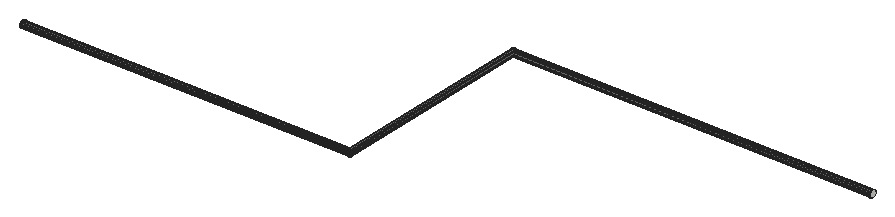
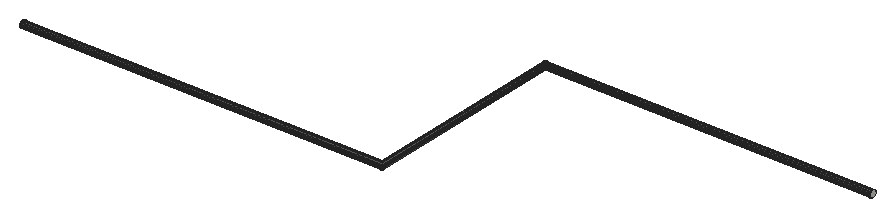
# SketchUp Ruby script. Lengths in inches.
U = 1.inch
M = Sketchup.active_model
def pt(a) = Geom::Point3d.new(a.map { |v| v * U })
def face(e, loops, mat)
  f = e.add_face(loops[0].map { |a| pt(a) })
  loops[1..].each { |l| e.add_face(l.map { |a| pt(a) }).erase! }
  f.material = f.back_material = mat if mat
  f
end
# faces: each face lists its corners as indices into pts; further lists are holes
def faces(e, pts, list, mat = nil) = list.each { |f| face(e, (f[0].is_a?(Array) ? f : [f]).map { |l| l.map { |i| pts[i] } }, mat) }
# xy, xz, yz: faces in a plane at the given z, y or x. An outline is a flat list of corners, or four numbers for a rectangle; further outlines are holes
def ring(l) = l.size == 4 ? [[l[0], l[1]], [l[2], l[1]], [l[2], l[3]], [l[0], l[3]]] : l.each_slice(2).to_a
def flat(e, list, mat, &to3) = list.each { |f| face(e, (f[0].is_a?(Array) ? f : [f]).map { |l| ring(l).map { |u, v| to3.(u, v) } }, mat) }
def xy(e, z, list, mat = nil) = flat(e, list, mat) { |x, y| [x, y, z] }
def xz(e, y, list, mat = nil) = flat(e, list, mat) { |x, z| [x, y, z] }
def yz(e, x, list, mat = nil) = flat(e, list, mat) { |y, z| [x, y, z] }
def lines(e, pts, list) = list.each { |a, b| e.add_line(pt(pts[a]), pt(pts[b])) }
# prism: a flat outline (further loops are holes) pulled along v
def prism(e, loops, v, mat = nil)
  f = face(e, loops, mat); d = Geom::Vector3d.new(v.map { |x| x * U })
  f.pushpull(f.normal.samedirection?(d) ? d.length : -d.length)
end
def box(e, o, s, mat = nil) = prism(e, [[o, [o[0] + s[0], o[1], o[2]], [o[0] + s[0], o[1] + s[1], o[2]], [o[0], o[1] + s[1], o[2]]]], [0, 0, s[2]], mat)
def at(x, y, z, deg = 0) = Geom::Transformation.translation(pt([x, y, z])) * Geom::Transformation.rotation(ORIGIN, Z_AXIS, deg.degrees)
def axes(o, x, y, z) = Geom::Transformation.new([*x, 0, *y, 0, *z, 0, *pt(o).to_a, 1])
def part(name) = M.definitions.add(name)
# library, detail: a bought-in or finely detailed component or shape, given as its bounding box
def library(name, o, s) = part(name).tap { |d| box(d.entities, o, s) }
def detail(e, o, s) = box(e.add_group.entities, o, s)
def put(e, d, t, mat = nil) = e.add_instance(d, t).tap { |i| i.material = mat if mat }
def group(e, t, mat = nil) = e.add_group.tap { |g| g.transformation = t; g.material = mat if mat }.entities
root = M.entities
M.materials.add("[Color M05]").color = [114, 114, 114]
yz(root,18,[[228,288.3125,227.74,288.34,227.5,288.44,227.29,288.6,227.13,288.8125,227.03,289.05,227,289.3125,227.03,289.57,227.13,289.8125,227.29,290.02,227.5,290.18,227.74,290.28,228,290.3125,228.26,290.28,228.5,290.18,228.71,290.02,228.87,289.8125,228.97,289.57,229,289.3125,228.97,289.05,228.87,288.8125,228.71,288.6,228.5,288.44,228.26,288.34]])
yz(root,231,[[291,288.3125,291.26,288.34,291.5,288.44,291.71,288.6,291.87,288.8125,291.97,289.05,292,289.3125,291.97,289.57,291.87,289.8125,291.71,290.02,291.5,290.18,291.26,290.28,291,290.3125,290.74,290.28,290.5,290.18,290.29,290.02,290.13,289.8125,290.03,289.57,290,289.3125,290.03,289.05,290.13,288.8125,290.29,288.6,290.5,288.44,290.74,288.34]])
p = [[119.76,227.74,288.34],[120,227.5,288.44],[18,227.5,288.44],[18,227.74,288.34],[119.76,290.74,288.34],[120,290.5,288.44],
  [119.5,228,288.3125],[18,228,288.3125],[119.5,291,288.3125],[119.24,228.26,288.34],[18,228.26,288.34],[119.24,291.26,288.34],
  [119,228.5,288.44],[18,228.5,288.44],[119,291.5,288.44],[231,290.74,288.34],[231,290.5,288.44],[231,291,288.3125],
  [231,291.26,288.34],[231,291.5,288.44],[120.21,227.29,288.6],[18,227.29,288.6],[120.21,290.29,288.6],[118.79,228.71,288.6],
  [18,228.71,288.6],[118.79,291.71,288.6],[231,290.29,288.6],[231,291.71,288.6],[120.37,227.13,288.8125],[18,227.13,288.8125],
  [120.37,290.13,288.8125],[118.63,228.87,288.8125],[18,228.87,288.8125],[118.63,291.87,288.8125],[231,290.13,288.8125],[231,291.87,288.8125],
  [120.47,227.03,289.05],[18,227.03,289.05],[120.47,290.03,289.05],[118.53,228.97,289.05],[18,228.97,289.05],[118.53,291.97,289.05],
  [231,290.03,289.05],[231,291.97,289.05],[120.5,227,289.3125],[18,227,289.3125],[120.5,290,289.3125],[118.5,229,289.3125],
  [18,229,289.3125],[118.5,292,289.3125],[231,290,289.3125],[231,292,289.3125],[120.47,227.03,289.57],[18,227.03,289.57],
  [120.47,290.03,289.57],[118.53,228.97,289.57],[18,228.97,289.57],[118.53,291.97,289.57],[231,290.03,289.57],[231,291.97,289.57],
  [120.37,227.13,289.8125],[18,227.13,289.8125],[120.37,290.13,289.8125],[118.63,228.87,289.8125],[18,228.87,289.8125],[118.63,291.87,289.8125],
  [231,290.13,289.8125],[231,291.87,289.8125],[120.21,227.29,290.02],[18,227.29,290.02],[120.21,290.29,290.02],[118.79,228.71,290.02],
  [18,228.71,290.02],[118.79,291.71,290.02],[231,290.29,290.02],[231,291.71,290.02],[120,227.5,290.18],[18,227.5,290.18],
  [120,290.5,290.18],[119,228.5,290.18],[18,228.5,290.18],[119,291.5,290.18],[231,290.5,290.18],[231,291.5,290.18],
  [119.76,227.74,290.28],[18,227.74,290.28],[119.76,290.74,290.28],[119.24,228.26,290.28],[18,228.26,290.28],[119.24,291.26,290.28],
  [231,290.74,290.28],[231,291.26,290.28],[119.5,228,290.3125],[18,228,290.3125],[119.5,291,290.3125],[231,291,290.3125]]
faces(root,p,[[0,1,2,3],[4,5,1,0],[6,0,3,7],[8,4,0,6],[9,6,7,10],[11,8,6,9],[12,9,10,13],[14,11,9,12],
  [15,16,5,4],[17,15,4,8],[18,17,8,11],[19,18,11,14],[1,20,21,2],[5,22,20,1],[23,12,13,24],[25,14,12,23],
  [16,26,22,5],[27,19,14,25],[20,28,29,21],[22,30,28,20],[31,23,24,32],[33,25,23,31],[26,34,30,22],[35,27,25,33],
  [28,36,37,29],[30,38,36,28],[39,31,32,40],[41,33,31,39],[34,42,38,30],[43,35,33,41],[36,44,45,37],[38,46,44,36],
  [47,39,40,48],[49,41,39,47],[42,50,46,38],[51,43,41,49],[44,52,53,45],[46,54,52,44],[55,47,48,56],[57,49,47,55],
  [50,58,54,46],[59,51,49,57],[52,60,61,53],[54,62,60,52],[63,55,56,64],[65,57,55,63],[58,66,62,54],[67,59,57,65],
  [60,68,69,61],[62,70,68,60],[71,63,64,72],[73,65,63,71],[66,74,70,62],[75,67,65,73],[68,76,77,69],[70,78,76,68],
  [79,71,72,80],[81,73,71,79],[74,82,78,70],[83,75,73,81],[76,84,85,77],[78,86,84,76],[87,79,80,88],[89,81,79,87],
  [82,90,86,78],[91,83,81,89],[84,92,93,85],[86,94,92,84],[92,87,88,93],[94,89,87,92],[90,95,94,86],[95,91,89,94]],"[Color M05]")
